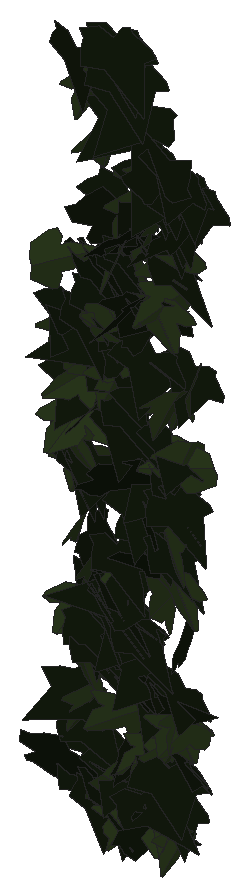
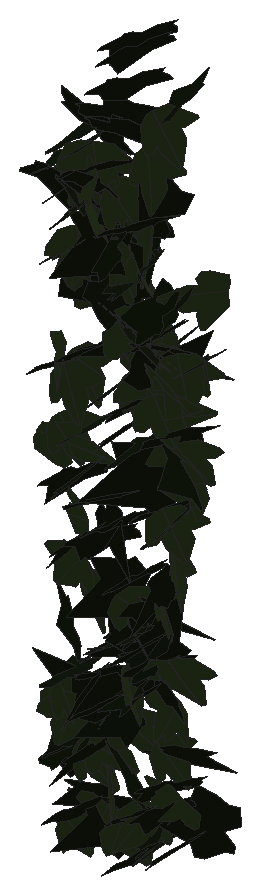
# SketchUp Ruby script. Lengths in inches.
U = 1.inch
M = Sketchup.active_model
def pt(a) = Geom::Point3d.new(a.map { |v| v * U })
def face(e, loops, mat)
  f = e.add_face(loops[0].map { |a| pt(a) })
  loops[1..].each { |l| e.add_face(l.map { |a| pt(a) }).erase! }
  f.material = f.back_material = mat if mat
  f
end
# faces: each face lists its corners as indices into pts; further lists are holes
def faces(e, pts, list, mat = nil) = list.each { |f| face(e, (f[0].is_a?(Array) ? f : [f]).map { |l| l.map { |i| pts[i] } }, mat) }
# xy, xz, yz: faces in a plane at the given z, y or x. An outline is a flat list of corners, or four numbers for a rectangle; further outlines are holes
def ring(l) = l.size == 4 ? [[l[0], l[1]], [l[2], l[1]], [l[2], l[3]], [l[0], l[3]]] : l.each_slice(2).to_a
def flat(e, list, mat, &to3) = list.each { |f| face(e, (f[0].is_a?(Array) ? f : [f]).map { |l| ring(l).map { |u, v| to3.(u, v) } }, mat) }
def xy(e, z, list, mat = nil) = flat(e, list, mat) { |x, y| [x, y, z] }
def xz(e, y, list, mat = nil) = flat(e, list, mat) { |x, z| [x, y, z] }
def yz(e, x, list, mat = nil) = flat(e, list, mat) { |y, z| [x, y, z] }
def lines(e, pts, list) = list.each { |a, b| e.add_line(pt(pts[a]), pt(pts[b])) }
# prism: a flat outline (further loops are holes) pulled along v
def prism(e, loops, v, mat = nil)
  f = face(e, loops, mat); d = Geom::Vector3d.new(v.map { |x| x * U })
  f.pushpull(f.normal.samedirection?(d) ? d.length : -d.length)
end
def box(e, o, s, mat = nil) = prism(e, [[o, [o[0] + s[0], o[1], o[2]], [o[0] + s[0], o[1] + s[1], o[2]], [o[0], o[1] + s[1], o[2]]]], [0, 0, s[2]], mat)
def at(x, y, z, deg = 0) = Geom::Transformation.translation(pt([x, y, z])) * Geom::Transformation.rotation(ORIGIN, Z_AXIS, deg.degrees)
def axes(o, x, y, z) = Geom::Transformation.new([*x, 0, *y, 0, *z, 0, *pt(o).to_a, 1])
def part(name) = M.definitions.add(name)
# library, detail: a bought-in or finely detailed component or shape, given as its bounding box
def library(name, o, s) = part(name).tap { |d| box(d.entities, o, s) }
def detail(e, o, s) = box(e.add_group.entities, o, s)
def put(e, d, t, mat = nil) = e.add_instance(d, t).tap { |i| i.material = mat if mat }
def group(e, t, mat = nil) = e.add_group.tap { |g| g.transformation = t; g.material = mat if mat }.entities
root = M.entities
M.materials.add("1026 AP 7946 SUNNY SIDE UP").color = [254, 231, 186]
M.materials.add("efeu1").color = [18, 25, 13]
M.materials.add("efeu2").color = [43, 57, 29]
c1 = part("ivyleaf_9")
p = [[1.54,2.16,1.25],[1.36,2.04,1.19],[-0.21,0.99,0.68],[-0.71,1.11,0.82],[-0.85,0.86,0.67],[-0.8,0.17,0.21],
  [-0.9,-0.01,0.1],[-0.67,-0.16,-0.02],[-0.08,-0.08,-0.05],[-0.03,-0.6,-0.4],[0.65,-0.88,-0.66],[0.83,-0.6,-0.49],
  [1.29,-0.42,-0.43],[1.8125,-0.07,-0.26],[1.21,0.44,0.15]]
faces(c1.entities,p,[[0,1,2,3,4,5,6,7,8,9,10,11,12,13,14]],"efeu1")
c2 = part("ivyleaf_10")
p = [[0,0.5,-0.03],[-0.0625,2.02,-0.43],[-0.19,2.01,-0.46],[-0.54,1.05,-0.29],[-0.52,0.625,-0.18],[-0.83,0.76,-0.28],
  [-1.16,0.64,-0.33],[-1.15,0.33,-0.24],[-0.77,-0.39,0.02],[-0.3,-0.51,0.16],[0.04,-0.48,0.23],[-0.02,2.01,-0.4375],
  [-0.06,2.01,-0.43],[0.04,-0.49,0.23],[0.67,-0.49,0.14],[1.38,0.36,-0.2],[1.375,0.51,-0.24],[0.81,0.65,-0.19],
  [0.62,0.59,-0.15],[0.6,1.09,-0.28],[0.5,1.23,-0.31]]
faces(c2.entities,p,[[0,1,2,3,4,5,6,7,8,9,10],[11,12,0,13,14,15,16,17,18,19,20]],"efeu2")
put(root,c1,axes([104.52,212.4,268.51],[0.27806,-0.01654,0.23802],[0.35145,-0.0646,-0.1813],[0.09621,0.28377,-0.02564]),"1026 AP 7946 SUNNY SIDE UP")
put(root,c2,axes([104.98,212.61,274.98],[-0.2551,-0.23777,0.02915],[-0.00638,-0.03307,-0.29632],[0.37671,-0.16157,0.01472]),"1026 AP 7946 SUNNY SIDE UP")
put(root,c2,axes([104.96,212.74,270.8],[0.37319,0.09535,-0.1094],[-0.15232,-0.04512,-0.2637],[-0.16566,0.25629,-0.00397]),"1026 AP 7946 SUNNY SIDE UP")
put(root,c2,axes([104.99,212.84,272.91],[-0.21301,-0.22749,0.08967],[-0.02228,-0.09353,-0.27107],[0.38308,-0.13193,0.03409]),"1026 AP 7946 SUNNY SIDE UP")
put(root,c1,axes([104.86,212.72,274.99],[-0.15934,-0.21805,0.17466],[-0.01887,-0.17822,-0.2428],[0.43509,-0.08759,0.05343]),"1026 AP 7946 SUNNY SIDE UP")
put(root,c2,axes([104.73,212.23,275.95],[0.01926,0.00017,-0.34037],[0.30569,0.26733,0.00913],[0.42006,-0.19455,0.00896]),"1026 AP 7946 SUNNY SIDE UP")
put(root,c1,axes([104.95,212.45,273.44],[0.14922,0.11886,0.26064],[0.07093,0.25648,-0.14045],[-0.4328,0.08302,0.06684]),"1026 AP 7946 SUNNY SIDE UP")
put(root,c1,axes([105.16,212.64,269.5],[-0.36646,-0.092,0.10465],[-0.12435,-0.07465,-0.25566],[0.17676,-0.24325,0.03712]),"1026 AP 7946 SUNNY SIDE UP")
put(root,c1,axes([104.81,212.8,278.85],[0.0444,-0.2684,0.15865],[0.00724,-0.15579,-0.27875],[0.48772,0.02675,-0.0103]),"1026 AP 7946 SUNNY SIDE UP")
put(root,c1,axes([105.03,212.79,274.06],[-0.23755,-0.22699,0.09405],[-0.03959,-0.09381,-0.27981],[0.38342,-0.15032,0.02938]),"1026 AP 7946 SUNNY SIDE UP")
put(root,c2,axes([104.83,212.56,273.37],[-0.26485,0.09815,-0.22149],[0.26169,-0.13916,-0.20006],[-0.265,-0.23552,0.02381]),"1026 AP 7946 SUNNY SIDE UP")
put(root,c2,axes([105.09,212.88,278.51],[-0.11562,-0.2789,0.108],[-0.00293,-0.10917,-0.29671],[0.46937,-0.06938,0.02475]),"1026 AP 7946 SUNNY SIDE UP")
put(root,c2,axes([105.125,212.59,274.25],[0.09876,0.07027,-0.29457],[-0.20251,-0.25682,-0.09553],[-0.41703,0.14135,-0.02337]),"1026 AP 7946 SUNNY SIDE UP")
put(root,c2,axes([105.09,212.45,273.69],[0.34323,0.141,-0.13851],[-0.16776,-0.08387,-0.26796],[-0.25737,0.24271,-0.01005]),"1026 AP 7946 SUNNY SIDE UP")
put(root,c2,axes([105.125,212.51,272.16],[0.05001,-0.26153,-0.1144],[-0.02818,0.10817,-0.27074],[0.44496,0.03624,-0.00429]),"1026 AP 7946 SUNNY SIDE UP")
put(root,c2,axes([105.13,212.86,274.47],[-0.25883,-0.21563,0.09713],[0.00643,-0.11906,-0.27037],[0.37077,-0.14846,0.07249]),"1026 AP 7946 SUNNY SIDE UP")
put(root,c1,axes([104.91,212.73,268.29],[0.09435,-0.24728,-0.06393],[0.00734,0.06337,-0.26104],[0.40029,0.05712,0.01986]),"1026 AP 7946 SUNNY SIDE UP")
put(root,c2,axes([104.87,212.8,268.96],[0.32785,-0.01326,0.17061],[0.2611,0.00475,-0.21485],[0.01167,0.26628,0.01389]),"1026 AP 7946 SUNNY SIDE UP")
put(root,c1,axes([104.95,212.72,272.88],[0.06423,-0.26614,0.09584],[0.01303,-0.09435,-0.27788],[0.44391,0.04128,-0.00571]),"1026 AP 7946 SUNNY SIDE UP")
put(root,c1,axes([104.91,212.81,275.89],[0.25777,-0.24831,-0.02958],[-0.02865,0.02069,-0.30638],[0.39175,0.1649,-0.00294]),"1026 AP 7946 SUNNY SIDE UP")
put(root,c1,axes([104.96,212.88,272.86],[0.06804,-0.26379,0.08793],[0.01235,-0.0867,-0.27583],[0.43652,0.04357,-0.0059]),"1026 AP 7946 SUNNY SIDE UP")
put(root,c2,axes([105.2,212.64,269.49],[-0.05326,-0.24139,0.12226],[-0.02342,-0.11913,-0.2518],[0.42326,-0.03697,0.00145]),"1026 AP 7946 SUNNY SIDE UP")
put(root,c1,axes([105.31,212.63,274.65],[0.10432,0.0748,0.29469],[-0.41793,-0.11236,0.09326],[0.20218,-0.27085,0.04072]),"1026 AP 7946 SUNNY SIDE UP")
put(root,c1,axes([105.05,212.87,268.83],[-0.02462,-0.25617,-0.06114],[0.0113,0.05756,-0.26403],[0.4128,-0.01685,0.00358]),"1026 AP 7946 SUNNY SIDE UP")
put(root,c1,axes([105.1875,212.61,271.92],[0.09102,-0.05031,-0.28139],[-0.24003,0.22698,-0.07515],[0.3643,0.16212,0.02079]),"1026 AP 7946 SUNNY SIDE UP")
put(root,c2,axes([105.14,212.57,270.08],[-0.36149,0.15011,-0.07455],[0.0735,-0.06176,-0.28201],[-0.25211,-0.23323,0.02468]),"1026 AP 7946 SUNNY SIDE UP")
put(root,c1,axes([105.01,212.69,269.125],[0.04775,-0.23244,-0.12419],[0.07454,0.12295,-0.23376],[0.40396,0.00479,0.05782]),"1026 AP 7946 SUNNY SIDE UP")
put(root,c2,axes([104.9375,212.9,274.72],[-0.05211,-0.05254,-0.29313],[0.32847,-0.20209,0.01221],[-0.31414,-0.2026,0.06139]),"1026 AP 7946 SUNNY SIDE UP")
put(root,c2,axes([105.1,212.5,274.96],[-0.38509,-0.06964,-0.14987],[0.24245,-0.02586,-0.2555],[0.07249,-0.28348,0.05835]),"1026 AP 7946 SUNNY SIDE UP")
put(root,c1,axes([105.1875,212.75,272.95],[-0.16122,-0.25759,0.07134],[0.01095,-0.07829,-0.28388],[0.41987,-0.09687,0.0348]),"1026 AP 7946 SUNNY SIDE UP")
put(root,c1,axes([105.14,212.78,270.5625],[-0.22007,-0.01078,-0.23807],[0.36073,-0.04073,-0.14145],[-0.04614,-0.26703,0.02959]),"1026 AP 7946 SUNNY SIDE UP")
put(root,c2,axes([105.33,212.76,277.82],[-0.12365,-0.2915,-0.05808],[0.02541,0.05232,-0.31073],[0.46567,-0.08026,0.00154]),"1026 AP 7946 SUNNY SIDE UP")
put(root,c2,axes([105.34,212.54,271.63],[0.05898,-0.28029,-0.02447],[-0.0014,0.02224,-0.29119],[0.44211,0.03746,0.00234]),"1026 AP 7946 SUNNY SIDE UP")
put(root,c1,axes([105.17,212.6,275.17],[0.04363,-0.2896,0.05455],[0.00895,-0.0543,-0.30003],[0.46331,0.02832,0.00066]),"1026 AP 7946 SUNNY SIDE UP")
put(root,c1,axes([105.64,212.52,274.9375],[-0.42347,-0.0347,0.14443],[-0.20469,-0.07112,-0.27577],[0.09907,-0.29527,0.04761]),"1026 AP 7946 SUNNY SIDE UP")
put(root,c1,axes([105.08,212.89,275.8],[0.23829,-0.23131,0.10342],[0.07651,-0.08966,-0.28529],[0.38987,0.15897,-0.00723]),"1026 AP 7946 SUNNY SIDE UP")
put(root,c1,axes([105.48,212.7,270.91],[0.23476,0.02482,0.23456],[-0.35884,-0.00486,0.15477],[0.02782,-0.27211,0.01702]),"1026 AP 7946 SUNNY SIDE UP")
put(root,c1,axes([105.22,212.79,275.41],[0.02465,-0.29248,0.00187],[0.01292,-0.00304,-0.30165],[0.45975,0.01577,0.00838]),"1026 AP 7946 SUNNY SIDE UP")
put(root,c1,axes([105.26,212.61,270.69],[-0.01522,-0.23939,-0.15606],[0.01283,0.14992,-0.24593],[0.44413,-0.01254,0.00175]),"1026 AP 7946 SUNNY SIDE UP")
put(root,c2,axes([105.51,212.61,276.64],[-0.27895,0.22218,0.11486],[-0.13909,0.06994,-0.29147],[-0.36434,-0.19681,0.02333]),"1026 AP 7946 SUNNY SIDE UP")
put(root,c2,axes([105.78,212.44,274.8125],[0.04263,0.00469,-0.30623],[-0.45234,0.07584,-0.02535],[0.11812,0.28872,0.01344]),"1026 AP 7946 SUNNY SIDE UP")
put(root,c1,axes([105.61,212.83,275.36],[-0.4012,0.09864,-0.09899],[0.10481,-0.08986,-0.27629],[-0.19018,-0.25762,0.05656]),"1026 AP 7946 SUNNY SIDE UP")
put(root,c1,axes([105.26,212.56,270.42],[0.11133,-0.25855,-0.07839],[0.01449,0.07945,-0.27411],[0.42289,0.06535,0.03003]),"1026 AP 7946 SUNNY SIDE UP")
put(root,c1,axes([105.34,212.59,268.07],[0.0067,-0.25104,0.07954],[0.00341,-0.07861,-0.25911],[0.41363,0.00472,0.00085]),"1026 AP 7946 SUNNY SIDE UP")
put(root,c2,axes([105.5,212.61,274.53],[-0.30549,-0.21405,-0.02095],[0.06744,-0.01336,-0.29492],[0.33112,-0.19476,0.04074]),"1026 AP 7946 SUNNY SIDE UP")
put(root,c1,axes([105.28,212.75,270.85],[0.22086,-0.19517,0.14272],[0.10125,-0.12522,-0.24776],[0.36352,0.15346,-0.0177]),"1026 AP 7946 SUNNY SIDE UP")
put(root,c1,axes([105.36,212.54,268.29],[0.20985,-0.25149,0.02934],[0.00381,-0.03254,-0.29318],[0.39821,0.13284,-0.01266]),"1026 AP 7946 SUNNY SIDE UP")
put(root,c1,axes([105.57,212.92,276.9],[-0.21056,-0.25782,0.07567],[0.01758,-0.089,-0.29547],[0.4218,-0.12499,0.05009]),"1026 AP 7946 SUNNY SIDE UP")
put(root,c2,axes([105.65,212.78,270.42],[0.05959,-0.26978,-0.00983],[0.00279,0.00833,-0.28059],[0.42438,0.03783,0.00322]),"1026 AP 7946 SUNNY SIDE UP")
put(root,c1,axes([105.51,212.8,270.89],[-0.04299,-0.26913,0.04632],[-0.00204,-0.04659,-0.27893],[0.42944,-0.02716,0.00331]),"1026 AP 7946 SUNNY SIDE UP")
put(root,c2,axes([105.76,212.65,275.2],[-0.29114,-0.19172,0.12618],[-0.09752,-0.11085,-0.27355],[0.34514,-0.19304,0.02915]),"1026 AP 7946 SUNNY SIDE UP")
put(root,c2,axes([105.7,212.78,271.48],[-0.15797,-0.15368,0.20814],[-0.01196,-0.21623,-0.17386],[0.40006,-0.06715,0.07699]),"1026 AP 7946 SUNNY SIDE UP")
put(root,c2,axes([105.68,212.6,274.51],[-0.12908,-0.25438,0.11386],[0.01264,-0.11887,-0.27284],[0.43683,-0.07172,0.04154]),"1026 AP 7946 SUNNY SIDE UP")
put(root,c1,axes([105.98,212.5,271.25],[-0.3708,0.03669,0.17132],[-0.26431,-0.00678,-0.24435],[-0.04096,-0.28836,0.02583]),"1026 AP 7946 SUNNY SIDE UP")
put(root,c1,axes([105.6,212.78,268.52],[-0.1669,-0.23105,0.07714],[-0.00216,-0.08256,-0.26037],[0.38255,-0.10127,0.03219]),"1026 AP 7946 SUNNY SIDE UP")
put(root,c2,axes([105.5625,212.54,268.43],[-0.1846,-0.178,-0.19977],[0.1786,0.15605,-0.21865],[0.37207,-0.16322,0.00584]),"1026 AP 7946 SUNNY SIDE UP")
put(root,c1,axes([105.42,212.84,276.27],[0.20474,-0.27076,-0.0122],[0.00298,0.01235,-0.30936],[0.42605,0.13003,0.00803]),"1026 AP 7946 SUNNY SIDE UP")
put(root,c1,axes([105.46,212.75,274.41],[0.06246,-0.27204,-0.08152],[0.04941,0.08211,-0.27952],[0.44205,0.02926,0.04276]),"1026 AP 7946 SUNNY SIDE UP")
put(root,c2,axes([105.64,212.64,276.27],[0.23803,-0.24331,0.10812],[0.05674,-0.10241,-0.29494],[0.41365,0.15406,-0.02176]),"1026 AP 7946 SUNNY SIDE UP")
put(root,c1,axes([105.6,212.86,267.93],[-0.05879,-0.24995,0.06494],[-0.01277,-0.06396,-0.26073],[0.40568,-0.03823,0.0012]),"1026 AP 7946 SUNNY SIDE UP")
put(root,c1,axes([105.47,212.64,271.17],[0.25549,-0.19975,-0.10808],[-0.00391,0.12639,-0.25389],[0.35392,0.14559,0.07522]),"1026 AP 7946 SUNNY SIDE UP")
put(root,c1,axes([105.875,212.8,278.1875],[-0.44638,-0.09862,0.039],[-0.03139,-0.0581,-0.30597],[0.16344,-0.28051,0.04775]),"1026 AP 7946 SUNNY SIDE UP")
put(root,c2,axes([105.96,212.48,269.57],[-0.24549,-0.09246,0.21625],[-0.26507,-0.12688,-0.18701],[0.2457,-0.22926,0.01431]),"1026 AP 7946 SUNNY SIDE UP")
put(root,c2,axes([105.63,212.52,275.36],[-0.38535,-0.11977,-0.10765],[0.18408,-0.00791,-0.27535],[0.16802,-0.26604,0.05478]),"1026 AP 7946 SUNNY SIDE UP")
put(root,c1,axes([105.53,212.72,270.31],[0.24926,-0.22126,-0.02505],[-0.03052,0.01445,-0.28022],[0.34846,0.15954,-0.00662]),"1026 AP 7946 SUNNY SIDE UP")
put(root,c1,axes([105.61,212.6875,279.32],[-0.02404,-0.30865,-0.05269],[0.01047,0.04912,-0.31805],[0.49139,-0.01615,0.0042]),"1026 AP 7946 SUNNY SIDE UP")
put(root,c1,axes([105.54,212.6,271.22],[0.23964,-0.24079,0.00557],[-0.0107,-0.01231,-0.29337],[0.37862,0.15206,-0.01182]),"1026 AP 7946 SUNNY SIDE UP")
put(root,c2,axes([105.69,212.82,276.35],[-0.33181,0.17774,-0.11614],[0.07886,-0.11401,-0.28005],[-0.3223,-0.21088,0.05105]),"1026 AP 7946 SUNNY SIDE UP")
put(root,c1,axes([105.58,212.71,276.13],[0.10789,-0.287,0.04832],[0.00379,-0.0493,-0.30414],[0.45767,0.06807,-0.00887]),"1026 AP 7946 SUNNY SIDE UP")
put(root,c1,axes([106,212.6,275.32],[-0.43035,0.09569,-0.03072],[0.02545,-0.04495,-0.29653],[-0.15579,-0.27167,0.03641]),"1026 AP 7946 SUNNY SIDE UP")
put(root,c1,axes([105.65,212.8,278.89],[-0.07912,-0.29833,-0.07666],[0.04036,0.06934,-0.31097],[0.48114,-0.05488,0.01348]),"1026 AP 7946 SUNNY SIDE UP")
put(root,c1,axes([105.63,212.64,271.83],[0.05324,-0.27251,-0.06155],[0.00557,0.05904,-0.28235],[0.43813,0.03236,0.01107]),"1026 AP 7946 SUNNY SIDE UP")
put(root,c1,axes([105.67,212.71,273.57],[-0.05704,-0.24528,0.15103],[0.01775,-0.15028,-0.25463],[0.4501,-0.02516,0.02918]),"1026 AP 7946 SUNNY SIDE UP")
put(root,c2,axes([105.66,212.69,271.09],[0.23429,-0.14158,0.18648],[0.18702,-0.13819,-0.21209],[0.31035,0.19016,-0.01297]),"1026 AP 7946 SUNNY SIDE UP")
put(root,c1,axes([105.625,212.23,273.02],[0.284,0.14929,0.21661],[0.2613,0.12755,-0.24059],[-0.30863,0.24537,-0.00437]),"1026 AP 7946 SUNNY SIDE UP")
put(root,c1,axes([105.65,212.71,274.01],[0.11892,-0.27077,-0.07763],[-0.0067,0.07533,-0.28873],[0.44125,0.07412,0.01654]),"1026 AP 7946 SUNNY SIDE UP")
put(root,c1,axes([105.97,212.24,276.7],[0.03529,0.30012,-0.02069],[-0.00223,-0.02174,-0.31018],[-0.47315,0.02249,-0.00008]),"1026 AP 7946 SUNNY SIDE UP")
put(root,c1,axes([105.68,212.51,279.41],[0.00426,-0.29949,-0.10024],[0.03325,0.09557,-0.30723],[0.49322,-0.00386,0.02158]),"1026 AP 7946 SUNNY SIDE UP")
put(root,c1,axes([105.65,212.5625,271.6],[0.32466,0.1356,0.14925],[0.2026,0.06594,-0.25371],[-0.23614,0.243,-0.01248]),"1026 AP 7946 SUNNY SIDE UP")
put(root,c1,axes([105.99,212.81,278.4],[-0.38962,-0.16833,0.05162],[-0.0385,-0.05435,-0.30729],[0.27391,-0.24709,0.03024]),"1026 AP 7946 SUNNY SIDE UP")
put(root,c1,axes([105.95,212.7,270.72],[-0.30895,-0.17689,0.07419],[-0.04948,-0.07337,-0.27075],[0.29682,-0.19635,0.03209]),"1026 AP 7946 SUNNY SIDE UP")
put(root,c2,axes([105.97,212.51,268.05],[-0.237,-0.17186,0.14463],[-0.04655,-0.15374,-0.22596],[0.34681,-0.13808,0.06851]),"1026 AP 7946 SUNNY SIDE UP")
put(root,c1,axes([105.7,212.73,274.64],[0.18886,-0.24244,-0.09925],[-0.0316,0.09564,-0.27716],[0.4082,0.11957,0.02446]),"1026 AP 7946 SUNNY SIDE UP")
put(root,c2,axes([105.96,212.64,277.07],[-0.06472,-0.27615,0.13427],[0.0022,-0.13326,-0.28774],[0.48121,-0.03653,0.01938]),"1026 AP 7946 SUNNY SIDE UP")
put(root,c1,axes([105.59,212.25,276.77],[0.07436,0.02834,0.34205],[0.50692,0.08034,-0.05392],[-0.13161,0.32545,-0.01444]),"1026 AP 7946 SUNNY SIDE UP")
put(root,c1,axes([105.81,212.43,268.68],[-0.06272,0.24329,0.12262],[0.01347,-0.11772,0.2531],[0.42471,0.03966,0.01008]),"1026 AP 7946 SUNNY SIDE UP")
put(root,c1,axes([106.18,212.54,272.46],[0.0472,0.04133,-0.29382],[-0.44505,0.05939,-0.02146],[0.08718,0.2808,0.04954]),"1026 AP 7946 SUNNY SIDE UP")
put(root,c2,axes([106.05,212.65,268.83],[0.12888,-0.22077,-0.13293],[-0.00847,0.13269,-0.23896],[0.40101,0.07376,0.03768]),"1026 AP 7946 SUNNY SIDE UP")
put(root,c1,axes([105.94,212.82,272.51],[-0.12195,-0.26647,0.06591],[-0.00344,-0.06745,-0.2858],[0.43145,-0.07586,0.01635]),"1026 AP 7946 SUNNY SIDE UP")
put(root,c1,axes([105.79,212.5625,269.82],[0.39037,-0.12262,0.01181],[0.00039,-0.02687,-0.28434],[0.19376,0.24711,-0.02323]),"1026 AP 7946 SUNNY SIDE UP")
put(root,c1,axes([106.1875,212.59,275.73],[-0.2144,0.14374,-0.23269],[0.09976,-0.22979,-0.19077],[-0.4101,-0.13105,0.07524]),"1026 AP 7946 SUNNY SIDE UP")
put(root,c1,axes([105.82,212.63,276.46],[0.44526,0.08742,0.08198],[0.12676,0.00651,-0.30477],[-0.13523,0.29393,-0.01575]),"1026 AP 7946 SUNNY SIDE UP")
put(root,c1,axes([105.85,212.82,276.47],[0.33561,-0.20712,-0.00405],[-0.02595,-0.01305,-0.30571],[0.32466,0.21306,-0.02024]),"1026 AP 7946 SUNNY SIDE UP")
put(root,c1,axes([106.16,212.96,272.83],[-0.26823,-0.18554,0.12163],[-0.0393,-0.13337,-0.25166],[0.34447,-0.1597,0.06601]),"1026 AP 7946 SUNNY SIDE UP")
put(root,c1,axes([105.96,212.57,270.81],[0.09934,-0.26113,-0.0863],[0.02605,0.08794,-0.27388],[0.42972,0.05504,0.03655]),"1026 AP 7946 SUNNY SIDE UP")
put(root,c1,axes([106.05,212.8,272.34],[-0.05546,-0.25972,-0.09977],[0.03674,0.093,-0.26928],[0.43349,-0.04111,0.01006]),"1026 AP 7946 SUNNY SIDE UP")
put(root,c1,axes([106.31,212.41,275.73],[0.23772,0.16472,-0.21475],[-0.18505,-0.1747,-0.23014],[-0.37582,0.19021,-0.02252]),"1026 AP 7946 SUNNY SIDE UP")
put(root,c1,axes([106.24,212.62,270.25],[-0.26857,-0.18536,0.09939],[-0.03998,-0.10657,-0.25515],[0.3269,-0.16532,0.05045]),"1026 AP 7946 SUNNY SIDE UP")
put(root,c2,axes([106.375,212.55,269.14],[-0.16211,-0.13284,0.21247],[-0.14184,-0.18838,-0.17193],[0.35979,-0.13412,0.02795]),"1026 AP 7946 SUNNY SIDE UP")
put(root,c2,axes([106.26,212.72,276.9],[0.10999,-0.28694,0.0662],[0.00503,-0.06698,-0.30439],[0.46291,0.06891,-0.01242]),"1026 AP 7946 SUNNY SIDE UP")
put(root,c2,axes([106.32,212.65,277.54],[-0.4131,-0.14198,0.04398],[-0.03831,-0.04598,-0.3065],[0.23032,-0.26229,0.0279]),"1026 AP 7946 SUNNY SIDE UP")
put(root,c1,axes([106.2,212.79,269.83],[-0.12589,-0.24181,0.09626],[-0.01601,-0.09622,-0.26222],[0.40809,-0.07837,0.01941]),"1026 AP 7946 SUNNY SIDE UP")
put(root,c1,axes([106.27,212.81,277.42],[-0.25762,-0.24168,0.08117],[-0.01374,-0.08993,-0.29824],[0.40014,-0.15869,0.04202]),"1026 AP 7946 SUNNY SIDE UP")
put(root,c1,axes([106.24,212.63,274.88],[-0.15997,-0.27036,0.04899],[-0.00909,-0.05023,-0.29762],[0.43197,-0.10118,0.01188]),"1026 AP 7946 SUNNY SIDE UP")
put(root,c1,axes([106.21,212.31,268.02],[0.03823,0.02542,-0.28057],[-0.02922,0.27308,0.02614],[0.42933,0.01632,0.02676]),"1026 AP 7946 SUNNY SIDE UP")
put(root,c1,axes([106.25,212.75,269.24],[0.13374,-0.20479,-0.15732],[-0.05314,0.14929,-0.22649],[0.39706,0.08896,0.02268]),"1026 AP 7946 SUNNY SIDE UP")
put(root,c2,axes([106.49,212.53,271.41],[0.27914,-0.15955,-0.16362],[-0.12027,0.14629,-0.23999],[0.33186,0.18722,0.05065]),"1026 AP 7946 SUNNY SIDE UP")
put(root,c1,axes([106.3125,212.66,270.11],[0.18109,-0.18569,-0.1649],[-0.15932,0.12371,-0.2237],[0.34984,0.15246,-0.01652]),"1026 AP 7946 SUNNY SIDE UP")
put(root,c2,axes([106.33,212.77,277.33],[-0.28609,0.22506,-0.08549],[0.07342,-0.07057,-0.29845],[-0.37067,-0.18768,0.00687]),"1026 AP 7946 SUNNY SIDE UP")
put(root,c2,axes([106.22,212.49,268.24],[0.41904,0.01978,0.11819],[0.18233,-0.02294,-0.27382],[-0.0142,0.28919,-0.0281]),"1026 AP 7946 SUNNY SIDE UP")
put(root,c2,axes([106.46,212.62,269.04],[-0.05347,-0.22836,0.13098],[-0.00219,-0.12936,-0.23808],[0.41197,-0.03032,0.01574]),"1026 AP 7946 SUNNY SIDE UP")
put(root,c1,axes([106.625,212.25,277.66],[0.15674,0.07048,0.28888],[-0.26823,0.25338,-0.00165],[-0.36632,-0.15538,0.12482]),"1026 AP 7946 SUNNY SIDE UP")
put(root,c2,axes([106.41,212.45,275.76],[-0.44337,-0.02513,-0.08081],[0.12848,-0.05411,-0.28556],[0.01458,-0.28759,0.05903]),"1026 AP 7946 SUNNY SIDE UP")
put(root,c1,axes([106.32,212.93,276.92],[0.01905,-0.28713,0.08761],[0.0032,-0.08666,-0.29656],[0.47159,0.01219,-0.00152]),"1026 AP 7946 SUNNY SIDE UP")
put(root,c1,axes([106.23,212.4375,268.43],[-0.00948,-0.15828,-0.21902],[0.26278,0.16178,-0.12856],[0.32202,-0.13668,0.09847]),"1026 AP 7946 SUNNY SIDE UP")
put(root,c2,axes([106.625,212.57,275.94],[-0.14334,-0.17871,0.22363],[-0.09944,-0.21041,-0.20609],[0.43206,-0.10772,0.02676]),"1026 AP 7946 SUNNY SIDE UP")
put(root,c2,axes([106.5,212.73,276.32],[-0.26874,-0.24145,-0.03897],[0.08659,0.00524,-0.30169],[0.37406,-0.17467,0.04184]),"1026 AP 7946 SUNNY SIDE UP")
put(root,c2,axes([106.59,212.81,274.38],[-0.11238,-0.28432,0.01587],[-0.00171,-0.01727,-0.3021],[0.44786,-0.07141,0.00283]),"1026 AP 7946 SUNNY SIDE UP")
put(root,c1,axes([106.37,212.82,273.08],[0.12707,-0.2758,-0.01823],[-0.00607,0.01568,-0.29598],[0.43437,0.0809,0.0012]),"1026 AP 7946 SUNNY SIDE UP")
put(root,c2,axes([106.87,212.76,273.38],[-0.13643,0.01476,0.28287],[-0.34416,-0.17786,-0.06246],[0.26151,-0.22637,0.06537]),"1026 AP 7946 SUNNY SIDE UP")
put(root,c1,axes([106.23,212.51,269.72],[0.06824,-0.03869,0.29576],[0.37566,-0.15979,-0.06028],[0.25822,0.24269,0.00953]),"1026 AP 7946 SUNNY SIDE UP")
put(root,c2,axes([106.65,212.49,274.43],[-0.07654,-0.28151,0.07886],[-0.01096,-0.07808,-0.2947],[0.45926,-0.04878,0.00611]),"1026 AP 7946 SUNNY SIDE UP")
put(root,c1,axes([106.49,212.77,273.58],[-0.10932,-0.24077,0.14781],[0.02713,-0.15259,-0.25366],[0.44098,-0.0503,0.05225]),"1026 AP 7946 SUNNY SIDE UP")
put(root,c1,axes([106.48,212.82,268.32],[-0.05215,-0.25901,-0.01121],[0.00837,0.00881,-0.26892],[0.40745,-0.03333,0.00409]),"1026 AP 7946 SUNNY SIDE UP")
put(root,c1,axes([106.79,212.57,277.04],[-0.36334,0.18385,-0.10968],[0.09398,-0.09627,-0.30252],[-0.32142,-0.23597,0.03553]),"1026 AP 7946 SUNNY SIDE UP")
put(root,c1,axes([106.38,212.72,276.38],[0.17509,-0.26575,-0.07658],[0.0041,0.07956,-0.29452],[0.43326,0.10665,0.03373]),"1026 AP 7946 SUNNY SIDE UP")
put(root,c1,axes([106.45,212.69,272.12],[0.10481,-0.25938,-0.09699],[-0.01979,0.09238,-0.27515],[0.43265,0.06706,0.01091]),"1026 AP 7946 SUNNY SIDE UP")
put(root,c1,axes([106.47,212.83,277.2],[0.03272,-0.29455,0.05168],[0.00402,-0.05178,-0.30451],[0.47026,0.02094,-0.00099]),"1026 AP 7946 SUNNY SIDE UP")
put(root,c1,axes([106.61,212.89,277.27],[-0.32686,-0.17816,-0.1324],[0.18294,0.05917,-0.28022],[0.2919,-0.23658,0.02736]),"1026 AP 7946 SUNNY SIDE UP")
put(root,c2,axes([106.72,212.7,273.61],[-0.12989,-0.25787,0.09806],[0.01639,-0.10376,-0.27663],[0.43271,-0.07348,0.03991]),"1026 AP 7946 SUNNY SIDE UP")
put(root,c1,axes([106.58,212.71,277.7],[-0.10385,-0.25239,0.16367],[0.01416,-0.16577,-0.26602],[0.46992,-0.05078,0.04419]),"1026 AP 7946 SUNNY SIDE UP")
put(root,c2,axes([106.72,212.59,267.92],[-0.06957,-0.22696,0.132],[0.02005,-0.13298,-0.23654],[0.41033,-0.03198,0.03394]),"1026 AP 7946 SUNNY SIDE UP")
put(root,c1,axes([106.625,212.98,274.67],[-0.14861,-0.25858,0.08265],[0.00109,-0.08674,-0.28254],[0.4264,-0.0899,0.02952]),"1026 AP 7946 SUNNY SIDE UP")
put(root,c1,axes([106.77,212.5,270.66],[0.07052,0.02519,0.30168],[0.05948,0.29312,-0.03025],[-0.45809,0.04194,0.04252]),"1026 AP 7946 SUNNY SIDE UP")
put(root,c2,axes([106.88,212.49,269.65],[-0.30657,-0.13161,0.13511],[-0.13219,-0.10824,-0.23991],[0.26147,-0.20903,0.03713]),"1026 AP 7946 SUNNY SIDE UP")
put(root,c2,axes([106.63,212.62,271.68],[-0.35669,0.09833,-0.13763],[0.14178,-0.11795,-0.24682],[-0.21977,-0.23568,0.06414]),"1026 AP 7946 SUNNY SIDE UP")
put(root,c2,axes([106.71,212.55,269.58],[-0.33919,-0.14675,-0.06783],[0.10619,0.0158,-0.26753],[0.22895,-0.22474,0.0236]),"1026 AP 7946 SUNNY SIDE UP")
put(root,c2,axes([106.58,212.57,272.27],[-0.15688,0.11016,-0.26124],[0.17075,-0.23302,-0.1493],[-0.40078,-0.1424,0.03865]),"1026 AP 7946 SUNNY SIDE UP")
put(root,c1,axes([106.58,212.88,277.52],[-0.02658,-0.28566,0.09548],[0.0523,-0.09564,-0.2929],[0.47011,-0.00551,0.03798]),"1026 AP 7946 SUNNY SIDE UP")
put(root,c2,axes([106.89,212.58,274.52],[0.00291,0.07068,0.29653],[-0.2657,0.23625,-0.05734],[-0.38213,-0.16373,0.04213]),"1026 AP 7946 SUNNY SIDE UP")
put(root,c1,axes([106.625,212.46,268.9375],[-0.12766,-0.25104,-0.09013],[0.07814,0.07403,-0.27031],[0.4099,-0.0923,0.02346]),"1026 AP 7946 SUNNY SIDE UP")
put(root,c2,axes([106.82,212.59,269.77],[-0.05157,-0.25323,0.09293],[0.00995,-0.09302,-0.263],[0.42334,-0.02866,0.0175]),"1026 AP 7946 SUNNY SIDE UP")
put(root,c1,axes([106.64,212.57,272.93],[0.01907,-0.25981,-0.12252],[0.01184,0.11781,-0.26698],[0.44818,0.00794,0.01227]),"1026 AP 7946 SUNNY SIDE UP")
put(root,c1,axes([106.68,212.7,270.07],[-0.09483,-0.22547,0.14606],[0.05469,-0.15205,-0.23266],[0.4163,-0.03138,0.06384]),"1026 AP 7946 SUNNY SIDE UP")
put(root,c1,axes([106.69,212.74,268.97],[-0.0607,-0.16312,0.21097],[0.10786,-0.20697,-0.15702],[0.39847,0.03117,0.07464]),"1026 AP 7946 SUNNY SIDE UP")
